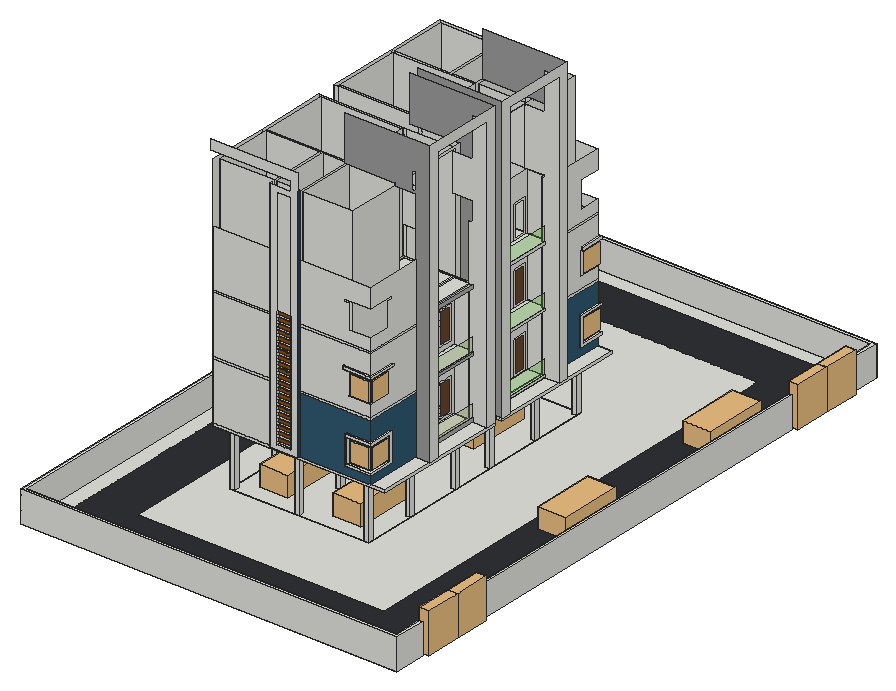
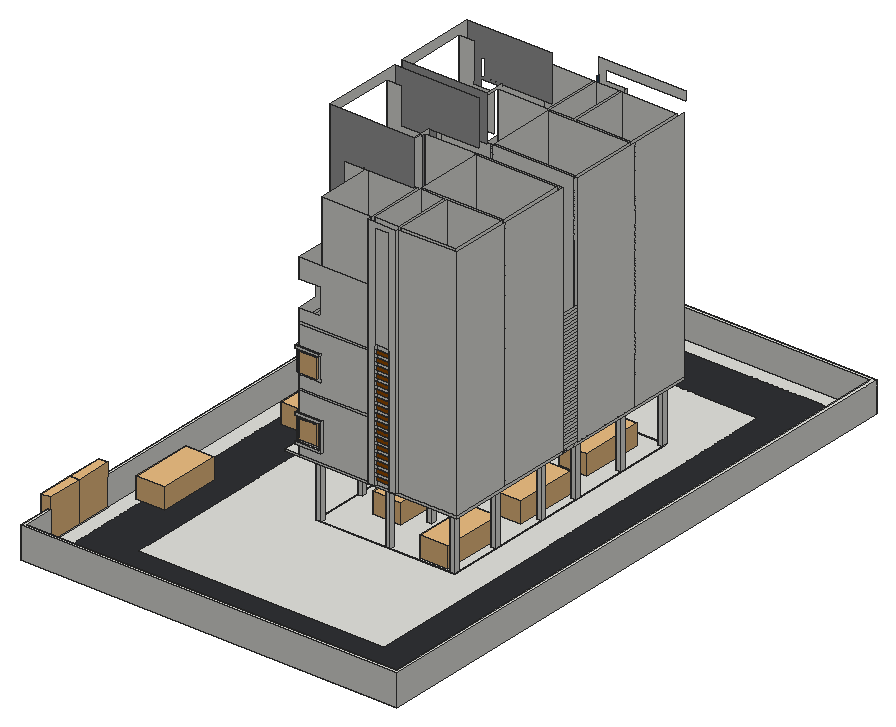
# SketchUp Ruby script. Lengths in inches.
U = 1.inch
M = Sketchup.active_model
def pt(a) = Geom::Point3d.new(a.map { |v| v * U })
def face(e, loops, mat)
  f = e.add_face(loops[0].map { |a| pt(a) })
  loops[1..].each { |l| e.add_face(l.map { |a| pt(a) }).erase! }
  f.material = f.back_material = mat if mat
  f
end
# faces: each face lists its corners as indices into pts; further lists are holes
def faces(e, pts, list, mat = nil) = list.each { |f| face(e, (f[0].is_a?(Array) ? f : [f]).map { |l| l.map { |i| pts[i] } }, mat) }
# xy, xz, yz: faces in a plane at the given z, y or x. An outline is a flat list of corners, or four numbers for a rectangle; further outlines are holes
def ring(l) = l.size == 4 ? [[l[0], l[1]], [l[2], l[1]], [l[2], l[3]], [l[0], l[3]]] : l.each_slice(2).to_a
def flat(e, list, mat, &to3) = list.each { |f| face(e, (f[0].is_a?(Array) ? f : [f]).map { |l| ring(l).map { |u, v| to3.(u, v) } }, mat) }
def xy(e, z, list, mat = nil) = flat(e, list, mat) { |x, y| [x, y, z] }
def xz(e, y, list, mat = nil) = flat(e, list, mat) { |x, z| [x, y, z] }
def yz(e, x, list, mat = nil) = flat(e, list, mat) { |y, z| [x, y, z] }
def lines(e, pts, list) = list.each { |a, b| e.add_line(pt(pts[a]), pt(pts[b])) }
# prism: a flat outline (further loops are holes) pulled along v
def prism(e, loops, v, mat = nil)
  f = face(e, loops, mat); d = Geom::Vector3d.new(v.map { |x| x * U })
  f.pushpull(f.normal.samedirection?(d) ? d.length : -d.length)
end
def box(e, o, s, mat = nil) = prism(e, [[o, [o[0] + s[0], o[1], o[2]], [o[0] + s[0], o[1] + s[1], o[2]], [o[0], o[1] + s[1], o[2]]]], [0, 0, s[2]], mat)
def at(x, y, z, deg = 0) = Geom::Transformation.translation(pt([x, y, z])) * Geom::Transformation.rotation(ORIGIN, Z_AXIS, deg.degrees)
def axes(o, x, y, z) = Geom::Transformation.new([*x, 0, *y, 0, *z, 0, *pt(o).to_a, 1])
def part(name) = M.definitions.add(name)
# library, detail: a bought-in or finely detailed component or shape, given as its bounding box
def library(name, o, s) = part(name).tap { |d| box(d.entities, o, s) }
def detail(e, o, s) = box(e.add_group.entities, o, s)
def put(e, d, t, mat = nil) = e.add_instance(d, t).tap { |i| i.material = mat if mat }
def group(e, t, mat = nil) = e.add_group.tap { |g| g.transformation = t; g.material = mat if mat }.entities
root = M.entities
M.materials.add("C07_Caramel_Shine").color = [153, 76, 0]
M.materials.add("Carpet_04_1K").color = [43, 65, 85]
M.materials.add("Glass_Basic_01").color = [173, 201, 98]
M.materials["Glass_Basic_01"].alpha = 0.25
M.materials.add("Glass_Basic_1").color = [130, 186, 66]
M.materials["Glass_Basic_1"].alpha = 0.25
M.materials.add("Glass_Basic_2").color = [93, 234, 42]
M.materials["Glass_Basic_2"].alpha = 0.25
M.materials.add("ThomThom - Buttons1").color = [48, 49, 53]
M.materials.add("ThomThom - Jumper1").color = [47, 89, 112]
M.materials.add("ThomThom - Waistcoat1").color = [155, 155, 155]
M.materials.add("ThomThom - Waistcoat2").color = [170, 170, 169]
M.materials.add("Wood_Veneer_15_1K").color = [103, 69, 45]
c1 = library("2016+Honda+Civic+LX+Sedan",[0.01,0.03,0.02],[16.17,34.46,10.62])
c2 = library("Ornamental gate leaf",[0,0,0],[161.42,42.43,280.3])
c3 = part("cong")
put(c3.entities,c2,axes([244.78,234.5625,0],[-1,0,0],[0,1,0],[0,0,1]))
put(c3.entities,c2,at(244.78,234.5625,0))
c4 = library("Group\#5",[0,0,0],[1.97,28.21,60])
xy(root,-12,[[[0,0,0,1506,948,1506,948,1421.02,939,1421.02,939,1241.02,948,1241.02,948,260.15,939,260.15,939,80.15,948,80.15,948,0],[240,360,588,1026]],[240,360,588,1026]])
xy(root,-6,[[[9,9,939,1497],[45,45,903,1461]],[[165,165,783,1341],[240,360,588,1026]],[240,360,588,1026]])
xy(root,-6,[[[45,45,903,1461],[165,165,783,1341]]],"ThomThom - Buttons1")
xy(root,66,[[0,0,948,0,948,80.15,939,80.15,939,9,9,9,9,1497,939,1497,939,1421.02,948,1421.02,948,1506,0,1506],[939,260.15,948,1241.02]])
xy(root,143.66,[[612,705,648,729],[612,885,648,909]])
xy(root,144,[[363,330,435,336],[[216,336,216,669,225,669,225,345,363,345,363,489,225,489,225,495,429,495,429,663,225,663,225,669,561,669,561,681,612,681,612,336],[435,495,555,663],[435,345,561,489],[369,345,429,489],[561,495,603,663]],[612,477,648,501],[612,657,648,681],[561,705,603,717],
  [555,723,561,891],[561,897,603,1041],[363,1050,381,1056],[417,1050,435,1056]])
xy(root,149.66,[[603,729,612,885]])
xy(root,155.71,[[381,1050,417,1053]])
xy(root,156,[[381,330,417,336]])
xy(root,163.125,[[381,333,417,336]])
xy(root,163.72,[[381,1050,417,1053]])
xy(root,168,[[552,330,558,336],[558,330,618,336],[612,336,618,337.15],[612,337.15,618,396],[612,990,618,1050],
  [551.39,1050,618,1056]])
xy(root,170.25,[[381,333,417,336]])
xy(root,172.65,[[381,1050,417,1053]])
xy(root,174,[[558,330,618,330,618,390,612,390,612,336,558,336],[612,996,612,1050,557.39,1050,557.39,1056,618,1056,618,996]])
xy(root,177.375,[[381,333,417,336]])
xy(root,181.57,[[381,1050,417,1053]])
xy(root,184.5,[[381,333,417,336]])
xy(root,190.5,[[381,1050,417,1053]])
xy(root,191.625,[[381,333,417,336]])
xy(root,198.75,[[381,333,417,336]])
xy(root,199.42,[[381,1050,417,1053]])
xy(root,205.875,[[381,333,417,336]])
xy(root,208.35,[[381,1050,417,1053]])
xy(root,213,[[381,333,417,336]])
xy(root,217.27,[[381,1050,417,1053]])
xy(root,220.125,[[381,333,417,336]])
xy(root,226.2,[[381,1050,417,1053]])
xy(root,227.25,[[381,333,417,336]])
xy(root,234,[[558,330,618,336],[612,336,618,390],[612,996,618,996,618,1056,557.39,1056,557.39,1050,612,1050]])
xy(root,234.375,[[381,333,417,336]])
xy(root,235.125,[[381,1050,417,1053]])
xy(root,240,[[552,330,618,330,618,396,612,396,612,336,552,336],[612,990,618,1050],[551.39,1050,618,1056]])
xy(root,241.5,[[381,333,417,336]])
xy(root,244.05,[[381,1050,417,1053]])
xy(root,248.625,[[381,333,417,336]])
xy(root,252.97,[[381,1050,417,1053]])
xy(root,255.75,[[381,333,417,336]])
xy(root,261.9,[[381,1050,417,1053]])
xy(root,262.875,[[381,333,417,336]])
xy(root,270,[[381,333,417,336]])
xy(root,270.82,[[381,1050,417,1053]])
xy(root,277.125,[[381,333,417,336]])
xy(root,279.75,[[381,1050,417,1053]])
xy(root,284.25,[[381,333,417,336]])
xy(root,288.67,[[381,1050,417,1053]])
xy(root,291.375,[[381,333,417,336]])
xy(root,293.66,[[435,723,555,891],[555,723,561,891],[561,723,603,723,603,729,612,729,612,885,603,885,603,891,561,891]])
xy(root,294,[[603,501,612,657]])
xy(root,297,[[435,495,555,501],[555,495,561,501],[561,495,603,501],[435,501,555,501.73],[555,501,561,501.73],
  [561,501,603,501.73],[435,501.73,555,657],[555,501.73,561,657],[561,501.73,603,657],[435,657,555,663],
  [555,657,561,663],[561,657,603,663]])
xy(root,297.6,[[381,1050,417,1053]])
xy(root,298.5,[[381,333,417,336]])
xy(root,299.66,[[435,723,555,891],[555,723,561,891],[561,723,561,891,603,891,603,885,612,885,612,729,603,729,603,723]])
xy(root,300,[[435,495,555,663],[555,495,561,663],[561,495,603,495,603,501,612,501,612,657,603,657,603,663,561,663],[603,495,612,501]])
xy(root,305.625,[[381,333,417,336]])
xy(root,306.52,[[381,1050,417,1053]])
xy(root,312.75,[[381,333,417,336]])
xy(root,315.45,[[381,1050,417,1053]])
xy(root,319.875,[[381,333,417,336]])
xy(root,324.375,[[381,1050,417,1053]])
xy(root,327,[[381,333,417,336]])
xy(root,333.3,[[381,1050,417,1053]])
xy(root,334.125,[[381,333,417,336]])
xy(root,341.25,[[381,333,417,336]])
xy(root,342.22,[[381,1050,417,1053]])
xy(root,348.375,[[381,333,417,336]])
xy(root,351.15,[[381,1050,417,1053]])
xy(root,355.5,[[381,333,417,336]])
xy(root,360.07,[[381,1050,417,1053]])
xy(root,362.625,[[381,333,417,336]])
xy(root,369,[[381,1050,417,1053]])
xy(root,369.75,[[381,333,417,336]])
xy(root,376.875,[[381,333,417,336]])
xy(root,377.92,[[381,1050,417,1053]])
xy(root,384,[[546,330,558,336],[558,330,612,336],[612,330,618,390],[381,333,417,336],[612,390,618,402],
  [612,996,618,1002],[612,1002,618,1056],[557.39,1050,564.01,1056],[564.01,1050,612,1056]])
xy(root,386.85,[[381,1050,417,1053]])
xy(root,390,[[546,330,618,330,618,402,612,402,612,336,546,336],[612,996,612,1050,557.39,1050,557.39,1056,618,1056,618,996]])
xy(root,391.125,[[381,333,417,336]])
xy(root,395.77,[[381,1050,417,1053]])
xy(root,398.25,[[381,333,417,336]])
xy(root,404.7,[[381,1050,417,1053]])
xy(root,405.375,[[381,333,417,336]])
xy(root,412.5,[[381,333,417,336]])
xy(root,413.625,[[381,1050,417,1053]])
xy(root,419.625,[[381,333,417,336]])
xy(root,422.55,[[381,1050,417,1053]])
xy(root,426.75,[[381,333,417,336]])
xy(root,431.47,[[381,1050,417,1053]])
xy(root,433.875,[[381,333,417,336]])
xy(root,440.4,[[381,1050,417,1053]])
xy(root,441,[[381,333,417,336]])
xy(root,443.66,[[435,723,555,891],[555,723,561,891],[561,723,603,723,603,729,612,729,612,885,603,885,603,891,561,891]])
xy(root,444,[[603,501,612,657]])
xy(root,448.125,[[381,333,417,336]])
xy(root,449.32,[[381,1050,417,1053]])
xy(root,449.66,[[435,723,555,891],[555,723,561,891],[561,723,561,891,603,891,603,885,612,885,612,729,603,729,603,723]])
xy(root,450,[[435,495,555,663],[555,495,561,663],[561,495,603,663]])
xz(root,0,[[0,-12,948,66]])
xz(root,9,[[9,-6,939,66]])
xz(root,80.15,[[939,-12,948,66]])
xz(root,260.15,[[939,-12,948,66]])
xz(root,330,[[[363,144,435,144,435,786,216,786,216,762,417,762,417,738,363,738],[381,156,417,726]],[552,168,618,168,618,174,558,174,558,234,618,234,618,240,552,240],[546,384,618,390]])
xz(root,333,[[381,163.125,417,170.25],[381,177.375,417,184.5],[381,191.625,417,198.75],[381,205.875,417,213],[381,220.125,417,227.25],
  [381,234.375,417,241.5],[381,248.625,417,255.75],[381,262.875,417,270],[381,277.125,417,284.25],[381,291.375,417,298.5],
  [381,305.625,417,312.75],[381,319.875,417,327],[381,334.125,417,341.25],[381,348.375,417,355.5],[381,362.625,417,369.75],
  [381,376.875,417,384],[381,391.125,417,398.25],[381,405.375,417,412.5],[381,419.625,417,426.75],[381,433.875,417,441],
  [381,448.125,417,455.25]],"C07_Caramel_Shine")
xz(root,336,[[216,144,363,288],[381,156,417,163.125],[381,170.25,417,177.375],[558,174,612,174,612,180,564,180,564,228,612,228,612,234,558,234],[564,180,612,228],
  [381,184.5,417,191.625],[381,198.75,417,205.875],[381,213,417,220.125],[381,227.25,417,234.375],[381,241.5,417,248.625],
  [381,255.75,417,262.875],[381,270,417,277.125],[381,284.25,417,291.375],[216,288,363,294],[435,288,612,294],
  [216,294,363,438],[435,294,612,294,612,324,558,324,558,384,546,384,546,390,612,390,612,438,435,438],[381,298.5,417,305.625],[381,312.75,417,319.875],[558,324,612,324,612,330,564,330,564,378,612,378,612,384,558,384],
  [381,327,417,334.125],[564,330,612,378],[381,341.25,417,348.375],[381,355.5,417,362.625],[381,369.75,417,376.875],
  [381,384,417,391.125],[381,398.25,417,405.375],[381,412.5,417,419.625],[381,426.75,417,433.875],[216,438,363,444],
  [435,438,612,444],[381,441,417,448.125],[216,444,363,588],[435,444,612,444,612,474,558,474,558,534,546,534,546,540,612,540,612,588,435,588]])
xz(root,336,[[435,144,612,144,612,168,552,168,552,240,612,240,612,288,435,288]],"ThomThom - Jumper1")
xz(root,345,[[225,144,363,738],[369,144,429,738],[435,144,561,738]])
xz(root,360,[[240,-12,588,-6]])
xz(root,390,[[612,174,618,234]])
xz(root,396,[[612,168,618,174],[612,174,618,234],[612,234,618,240]])
xz(root,402,[[612,384,618,390]])
xz(root,477,[[612,144,648,144,648,858,435,858,435,744,602.94,744,602.94,786,612,786,612,744,561,744,561,738,612,738]],"ThomThom - Waistcoat1")
xz(root,489,[[225,144,363,738],[369,144,429,738],[435,144,561,738]])
xz(root,495,[[225,144,429,738],[429,144,435,150],[435,144,555,297],[555,144,561,297],[561,144,603,297],
  [429,150,435,294],[429,294,435,300],[429,300,435,444],[435,300,555,450],[555,300,561,450],
  [561,300,603,450],[429,444,435,450],[429,450,435,594],[435,450,603,453]])
xz(root,501,[[612,144,612,150,603,150,603,294,612,294,612,300,603,300,603,444,612,444,612,453,603,453,603,594,612,594,612,642,561,642,561,738,613,738,613,744,612,744,612,834,648,834,648,144]])
xz(root,657,[[612,144,648,144,648,834,612,834,612,744,613,744,613,738,561,738,561,642,612,642,612,594,603,594,603,453,612,453,612,444,603,444,603,300,612,300,612,294,603,294,603,150,612,150]])
xz(root,663,[[225,144,429,738],[435,144,555,297],[561,144,603,297],[435,297,555,300],[555,297,561,300],
  [435,300,555,450],[561,300,603,450],[435,450,555,453],[555,450,561,453],[561,450,603,453]])
xz(root,669,[[216,144,225,738],[225,144,429,738],[429,144,435,738],[435,144,561,738]])
xz(root,681,[[561,144,561,744,435,744,435,858,648,858,648,144]],"ThomThom - Waistcoat1")
xz(root,705,[[612,143.66,612,144,561,144,561,744,435,744,435,858,648,858,648,143.66]],"ThomThom - Waistcoat1")
xz(root,717,[[216,144,225,738],[225,144,429,738],[429,144,435,738],[435,144,561,738]])
xz(root,723,[[225,144,429,738],[435,144,555,293.66],[555,144,561,293.66],[561,144,603,293.66],[435,293.66,603,299.66],
  [435,299.66,555,443.66],[555,299.66,561,443.66],[561,299.66,603,443.66],[435,443.66,603,449.66],[435,449.66,555,593.66],
  [555,449.66,561,593.66],[561,449.66,603,593.66]])
xz(root,729,[[612,143.66,648,143.66,648,834,612,834,612,743.66,561,743.66,561,599.66,612,599.66,612,593.66,603,593.66,603,449.66,612,449.66,612,443.66,603,443.66,603,299.66,612,299.66,612,293.66,603,293.66,603,149.66,612,149.66],[603,293.66,612,299.66],[603,443.66,612,449.66]])
xz(root,885,[[612,143.66,612,149.66,603,149.66,603,293.66,612,293.66,612,299.66,603,299.66,603,443.66,612,443.66,612,449.66,603,449.66,603,593.66,612,593.66,612,599.66,561,599.66,561,743.66,612,743.66,612,834,648,834,648,143.66],[603,293.66,612,299.66],[603,443.66,612,449.66]])
xz(root,891,[[225,144,429,738],[429,144,435,150],[435,144,555,293.66],[561,144,603,293.66],[429,150,435,294],
  [435,293.66,555,299.43],[555,293.66,561,299.43],[561,293.66,603,299.43],[429,294,435,300],[435,299.43,555,299.66],
  [555,299.43,561,299.66],[561,299.43,603,299.66],[435,299.66,555,443.66],[561,299.66,603,443.66],[429,300,435,444],
  [435,443.66,555,449.66],[555,443.66,561,449.66],[561,443.66,603,449.66],[429,444,435,450],[435,449.66,555,593.66],
  [561,449.66,603,593.66],[429,450,435,594]])
xz(root,897,[[225,144,363,738],[369,144,429,738],[435,144,561,738]])
xz(root,909,[[612,143.66,648,143.66,648,858,435,858,435,744,612,744]],"ThomThom - Waistcoat1")
xz(root,990,[[612,168,618,240]])
xz(root,996,[[612,174,618,234],[612,384,618,390]])
xz(root,1026,[[240,-12,588,-6]])
xz(root,1041,[[225,144,363,738],[369,144,429,738],[435,144,561,738]])
xz(root,1050,[[216,144,363,738],[381,144,417,155.71],[435,144,612,144,612,168,551.39,168,551.39,240,612,240,612,288,435,288],[381,163.72,417,172.65],[557.39,174,612,174,612,180,564.01,180,564.01,228,612,228,612,234,557.39,234],
  [564.01,180,612,228],[381,181.57,417,190.5],[381,199.42,417,208.35],[381,217.27,417,226.2],[381,235.125,417,244.05],
  [381,252.97,417,261.9],[381,270.82,417,279.75],[435,288,612,294],[381,288.67,417,297.6],[435,294,612,294,612,324,557.39,324,557.39,390,612,390,612,438,435,438],
  [381,306.52,417,315.45],[557.39,324,612,324,612,330,564.01,330,564.01,378,612,378,612,384,557.39,384],[381,324.375,417,333.3],[564.01,330,612,378],[381,342.22,417,351.15],
  [381,360.07,417,369],[381,377.92,417,386.85],[381,395.77,417,404.7],[381,413.625,417,422.55],[381,431.47,417,440.4],
  [435,438,612,444],[435,444,612,444,612,474,557.39,474,557.39,540,612,540,612,588,435,588],[381,449.32,417,458.25]])
xz(root,1053,[[381,155.71,417,163.72],[381,172.65,417,181.57],[381,190.5,417,199.42],[381,208.35,417,217.27],[381,226.2,417,235.125],
  [381,244.05,417,252.97],[381,261.9,417,270.82],[381,279.75,417,288.67],[381,297.6,417,306.52],[381,315.45,417,324.375],
  [381,333.3,417,342.22],[381,351.15,417,360.07],[381,369,417,377.92],[381,386.85,417,395.77],[381,404.7,417,413.625],
  [381,422.55,417,431.47],[381,440.4,417,449.32]],"C07_Caramel_Shine")
xz(root,1056,[[363,144,381,144,381,726,417,726,417,144,435,144,435,738,363,738],[551.39,168,618,168,618,174,557.39,174,557.39,234,618,234,618,240,551.39,240],[557.39,384,618,390]])
xz(root,1241.02,[[939,-12,948,66]])
xz(root,1421.02,[[939,-12,948,66]])
xz(root,1497,[[9,-6,939,66]])
xz(root,1506,[[0,-12,948,66]])
yz(root,0,[[0,-12,1506,66]])
yz(root,9,[[9,-6,1497,66]])
yz(root,216,[[669,138,717,145.5],[336,144,489,738],[489,144,669,738],[717,144,897,738],[897,144,1050,738],
  [669,145.5,717,153],[669,153,717,160.5],[669,160.5,717,168],[669,168,717,175.5],[669,175.5,717,183],
  [669,183,717,190.5],[669,190.5,717,198],[669,198,717,205.5],[669,205.5,717,213],[669,213,717,220.5],
  [669,220.5,717,228],[669,228,717,235.5],[669,235.5,717,243],[669,243,717,250.5],[669,250.5,717,258],
  [669,258,717,265.5],[669,265.5,717,273],[669,273,717,280.5],[669,280.5,717,288],[669,288,717,295.5],
  [669,295.5,717,303],[669,303,717,310.5],[669,310.5,717,318],[669,318,717,325.5],[669,325.5,717,333],
  [669,333,717,340.5],[669,340.5,717,348],[669,348,717,355.5],[669,355.5,717,363],[669,363,717,370.5],
  [669,370.5,717,378],[669,378,717,385.5],[669,385.5,717,393],[669,393,717,400.5],[669,400.5,717,408],
  [669,408,717,415.5],[669,415.5,717,423],[669,423,717,430.5],[669,430.5,717,438],[669,438,717,445.5],
  [669,445.5,717,453]])
yz(root,225,[[345,144,489,738],[489,144,495,150],[495,144,663,738],[663,144,669,150],[717,144,723,150],
  [723,144,891,738],[891,144,897,150],[897,144,1041,738],[489,150,495,294],[663,150,669,294],
  [717,150,723,294],[891,150,897,294],[489,294,495,300],[663,294,669,300],[717,294,723,300],
  [891,294,897,300],[489,300,495,444],[663,300,669,444],[717,300,723,444],[891,300,897,444],
  [489,444,495,450],[663,444,669,450],[717,444,723,450],[891,444,897,450],[489,450,495,594],
  [663,450,669,594],[717,450,723,594],[891,450,897,594]])
yz(root,240,[[360,-12,720,-6],[720,-12,1026,-6]])
yz(root,363,[[330,144,336,738],[345,144,489,738],[897,144,1041,738],[1050,144,1056,738]])
yz(root,369,[[345,144,489,738],[897,144,1041,738]])
yz(root,381,[[1050,144,1050,155.71,1053,155.71,1053,163.72,1056,163.72,1056,144],[330,156,336,163.125],[330,163.125,333,170.25],[1050,163.72,1056,172.65],[330,170.25,336,177.375],
  [1053,172.65,1056,181.57],[330,177.375,333,184.5],[1050,181.57,1056,190.5],[330,184.5,336,191.625],[1053,190.5,1056,199.42],
  [330,191.625,333,198.75],[330,198.75,336,205.875],[1050,199.42,1056,208.35],[330,205.875,333,213],[1053,208.35,1056,217.27],
  [330,213,336,220.125],[1050,217.27,1056,226.2],[330,220.125,333,227.25],[1053,226.2,1056,235.125],[330,227.25,336,234.375],
  [330,234.375,333,241.5],[1050,235.125,1056,244.05],[330,241.5,336,248.625],[1053,244.05,1056,252.97],[330,248.625,333,255.75],
  [1050,252.97,1056,261.9],[330,255.75,336,262.875],[1053,261.9,1056,270.82],[330,262.875,333,270],[330,270,336,277.125],
  [1050,270.82,1056,279.75],[330,277.125,333,284.25],[1053,279.75,1056,288.67],[330,284.25,336,291.375],[1050,288.67,1056,297.6],
  [330,291.375,333,298.5],[1053,297.6,1056,306.52],[330,298.5,336,305.625],[330,305.625,333,312.75],[1050,306.52,1056,315.45],
  [330,312.75,336,319.875],[1053,315.45,1056,324.375],[330,319.875,333,327],[1050,324.375,1056,333.3],[330,327,336,334.125],
  [1053,333.3,1056,342.22],[330,334.125,333,341.25],[330,341.25,336,348.375],[1050,342.22,1056,351.15],[330,348.375,333,355.5],
  [1053,351.15,1056,360.07],[330,355.5,336,362.625],[1050,360.07,1056,369],[330,362.625,333,369.75],[1053,369,1056,377.92],
  [330,369.75,336,376.875],[330,376.875,333,384],[1050,377.92,1056,386.85],[330,384,336,391.125],[1053,386.85,1056,395.77],
  [330,391.125,333,398.25],[1050,395.77,1056,404.7],[330,398.25,336,405.375],[1053,404.7,1056,413.625],[330,405.375,333,412.5],
  [330,412.5,336,419.625],[1050,413.625,1056,422.55],[330,419.625,333,426.75],[1053,422.55,1056,431.47],[330,426.75,336,433.875],
  [1050,431.47,1056,440.4],[330,433.875,333,441],[1053,440.4,1056,449.32],[330,441,336,448.125],[330,448.125,333,455.25],
  [1050,449.32,1056,458.25]])
yz(root,417,[[1050,144,1056,144,1056,163.72,1053,163.72,1053,155.71,1050,155.71],[330,156,336,163.125],[330,163.125,333,170.25],[1050,163.72,1056,172.65],[330,170.25,336,177.375],
  [1053,172.65,1056,181.57],[330,177.375,333,184.5],[1050,181.57,1056,190.5],[330,184.5,336,191.625],[1053,190.5,1056,199.42],
  [330,191.625,333,198.75],[330,198.75,336,205.875],[1050,199.42,1056,208.35],[330,205.875,333,213],[1053,208.35,1056,217.27],
  [330,213,336,220.125],[1050,217.27,1056,226.2],[330,220.125,333,227.25],[1053,226.2,1056,235.125],[330,227.25,336,234.375],
  [330,234.375,333,241.5],[1050,235.125,1056,244.05],[330,241.5,336,248.625],[1053,244.05,1056,252.97],[330,248.625,333,255.75],
  [1050,252.97,1056,261.9],[330,255.75,336,262.875],[1053,261.9,1056,270.82],[330,262.875,333,270],[330,270,336,277.125],
  [1050,270.82,1056,279.75],[330,277.125,333,284.25],[1053,279.75,1056,288.67],[330,284.25,336,291.375],[1050,288.67,1056,297.6],
  [330,291.375,333,298.5],[1053,297.6,1056,306.52],[330,298.5,336,305.625],[330,305.625,333,312.75],[1050,306.52,1056,315.45],
  [330,312.75,336,319.875],[1053,315.45,1056,324.375],[330,319.875,333,327],[1050,324.375,1056,333.3],[330,327,336,334.125],
  [1053,333.3,1056,342.22],[330,334.125,333,341.25],[330,341.25,336,348.375],[1050,342.22,1056,351.15],[330,348.375,333,355.5],
  [1053,351.15,1056,360.07],[330,355.5,336,362.625],[1050,360.07,1056,369],[330,362.625,333,369.75],[1053,369,1056,377.92],
  [330,369.75,336,376.875],[330,376.875,333,384],[1050,377.92,1056,386.85],[330,384,336,391.125],[1053,386.85,1056,395.77],
  [330,391.125,333,398.25],[1050,395.77,1056,404.7],[330,398.25,336,405.375],[1053,404.7,1056,413.625],[330,405.375,333,412.5],
  [330,412.5,336,419.625],[1050,413.625,1056,422.55],[330,419.625,333,426.75],[1053,422.55,1056,431.47],[330,426.75,336,433.875],
  [1050,431.47,1056,440.4],[330,433.875,333,441],[1053,440.4,1056,449.32],[330,441,336,448.125],[330,448.125,333,455.25],
  [1050,449.32,1056,458.25]])
yz(root,429,[[345,144,489,738],[495,144,663,738],[723,144,891,738],[897,144,1041,738]])
yz(root,435,[[345,144,489,738],[495,144,663,297],[723,144,891,293.66],[897,144,1041,738],[1050,144,1056,738],
  [495,297,663,300],[723,299.66,891,443.66],[495,300,663,450],[723,449.66,891,593.66],[495,450,663,453]])
yz(root,435,[[330,144,336,744]],"Carpet_04_1K")
yz(root,546,[[330,384,336,390]])
yz(root,551.39,[[1050,168,1056,240]])
yz(root,552,[[330,168,336,174],[330,174,336,234],[330,234,336,240]])
yz(root,557.39,[[1050,174,1056,234],[1050,384,1056,390]])
yz(root,558,[[330,174,336,234]])
yz(root,561,[[345,144,345,738,477,738,477,744,681,744,681,144,669,144,669,738,489,738,489,144],[[495,144,663,297],[615,148.61,651,232.61],[543,181.61,591,229.61]],[705,144,717,144,717,738,729,738,729,743.66,885,743.66,885,738,897,738,897,144,1041,144,1041,738,909,738,909,744,705,744],[[723,144,723,293.66,891,293.66,891,144,885,144,885,228,849,228,849,144],[777,180,825,228]],[[849,144,885,228],[852,147,882,225]],
  [[615,148.61,651,232.61],[618,151.61,648,229.61]],[[777,180,825,228],[780,183,822,225]],[[543,181.61,591,229.61],[546,184.61,588,226.61]],[[723,299.66,723,443.66,891,443.66,891,299.66,885,299.66,885,383.66,849,383.66,849,299.66],[777,335.66,825,383.66]],[[849,299.66,885,383.66],[852,302.66,882,380.66]],
  [[495,300,663,450],[615,311.08,651,395.08],[543,347.08,591,395.08]],[[615,311.08,651,395.08],[618,314.08,648,392.08]],[[777,335.66,825,383.66],[780,338.66,822,380.66]],[[543,347.08,591,395.08],[546,350.08,588,392.08]],[[723,449.66,723,593.66,891,593.66,891,449.66,885,449.66,885,533.66,849,533.66,849,449.66],[777,485.66,825,533.66]],
  [[849,449.66,885,533.66],[852,452.66,882,530.66]]])
yz(root,561,[[852,147,882,225],[618,151.61,648,229.61],[852,302.66,882,380.66],[618,314.08,648,392.08]],"Wood_Veneer_15_1K")
yz(root,588,[[360,-12,1026,-6]])
yz(root,603,[[[495,144,663,297],[501,150,657,294]],[723,144,891,144,891,293.66,885,293.66,885,149.66,729,149.66,729,293.66,723,293.66],[723,293.66,729,299.66],[885,293.66,891,299.43],[885,299.43,891,299.66],
  [723,299.66,729,443.66],[885,299.66,891,443.66],[495,300,495,450,663,450,663,300,657,300,657,444,501,444,501,300],[723,443.66,729,449.66],[885,443.66,891,449.66],
  [723,449.66,729,593.66],[885,449.66,891,593.66],[495,450,657,453],[657,450,663,453]])
yz(root,612,[[705,143.66,729,144],[729,143.66,885,144],[885,143.66,909,144],[729,144,885,149.66],[336,174,390,174,390,234,336,234,336,228,384,228,384,180,336,180],
  [996,174,996,234,1050,234,1050,228,1002,228,1002,180,1050,180,1050,174],[336,180,384,228],[1002,180,1050,228],[336,288,477,294],[909,288,1050,294],
  [729,293.66,885,299.66],[336,294,477,294,477,438,336,438,336,390,402,390,402,384,390,384,390,324,336,324],[909,294,909,438,1050,438,1050,390,996,390,996,324,1050,324,1050,294],[336,324,390,324,390,384,336,384,336,378,384,378,384,330,336,330],[996,324,996,384,1050,384,1050,378,1002,378,1002,330,1050,330,1050,324],
  [336,330,384,378],[1002,330,1050,378],[336,438,477,444],[909,438,1050,444],[729,443.66,885,449.66],
  [336,444,477,444,477,588,336,588,336,540,402,540,402,534,390,534,390,474,336,474],[909,444,909,588,1050,588,1050,540,996,540,996,474,1050,474,1050,444]])
yz(root,612,[[501,153,657,186]],"Glass_Basic_01")
yz(root,612,[[501,303,657,336]],"Glass_Basic_1")
yz(root,612,[[729,149.66,885,185.66],[729,299.66,885,335.66],[729,449.66,885,485.66]],"Glass_Basic_2")
yz(root,612,[[336,144,477,144,477,288,336,288,336,240,396,240,396,168,336,168],[909,144,909,288,1050,288,1050,240,990,240,990,168,1050,168,1050,144]],"ThomThom - Jumper1")
yz(root,612,[[501,144,657,153],[501,294,657,300],[501,300,657,303],[501,444,657,453]],"ThomThom - Waistcoat2")
yz(root,618,[[330,168,396,168,396,240,330,240,330,234,390,234,390,174,330,174],[990,168,990,240,1056,240,1056,234,996,234,996,174,1056,174,1056,168],[330,384,402,390],[996,384,1056,390]])
yz(root,648,[[705,143.66,705,858,909,858,909,143.66,885,143.66,885,834,729,834,729,143.66],[477,144,501,144,501,834,657,834,657,144,681,144,681,858,477,858]])
yz(root,939,[[80.15,-12,260.15,-6],[1241.02,-12,1421.02,-6],[9,-6,80.15,66],[260.15,-6,1241.02,66],[1421.02,-6,1497,66]])
yz(root,948,[[0,-12,80.15,66],[260.15,-12,1241.02,66],[1421.02,-12,1506,66]])
p = [[561,489,144],[612,489,144],[603,489,150],[612,489,150],[603,489,294],[612,489,294],
  [603,489,300],[612,489,300],[603,663,444],[612,663,444],[612,409.46,240],[558,336,240],
  [603,897,144],[612,897,144],[603,897,150],[612,897,150],[603,897,294],[612,897,294],
  [603,897,300],[612,897,300],[603,723,444],[612,723,444]]
lines(root,p,[[0,1],[2,3],[4,5],[6,7],[8,9],[10,11],[12,13],[14,15],[16,17],[18,19],[20,21]])
put(root,c1,axes([811.18,612.07,-8.65],[4.4275,0,0],[0,4.5484,0],[0,0,4.833]))
g1 = group(root,at(216,717,138))
xy(g1,-144,[[24,24,36,36],[186,24,198,36],[360,24,372,36],[24,166.5,36,178.5],[186,166.5,198,178.5],
  [360,166.5,372,178.5],[24,297,36,309],[186,297,198,309],[360,297,372,309]])
xy(g1,0,[[[0,-12,432,333],[24,24,372,309]],[36,24,186,36],[198,24,360,36],[24,36,36,166.5],[36,36,186,166.5],
  [186,36,198,166.5],[198,36,360,166.5],[360,36,372,166.5],[36,166.5,186,178.5],[198,166.5,360,178.5],
  [24,178.5,36,297],[36,178.5,186,297],[186,178.5,198,297],[198,178.5,360,297],[360,178.5,372,297],
  [36,297,186,309],[198,297,360,309]])
xy(g1,6,[[0,-12,432,333]])
xz(g1,-12,[[0,0,432,6]])
xz(g1,24,[[24,-144,36,0],[186,-144,198,0],[360,-144,372,0]])
xz(g1,36,[[24,-144,36,0],[186,-144,198,0],[360,-144,372,0]])
xz(g1,166.5,[[24,-144,36,0],[186,-144,198,0],[360,-144,372,0]])
xz(g1,178.5,[[24,-144,36,0],[186,-144,198,0],[360,-144,372,0]])
xz(g1,297,[[24,-144,36,0],[186,-144,198,0],[360,-144,372,0]])
xz(g1,309,[[24,-144,36,0],[186,-144,198,0],[360,-144,372,0]])
xz(g1,333,[[0,0,432,6]])
yz(g1,0,[[-12,0,333,6]])
yz(g1,24,[[24,-144,36,0],[166.5,-144,178.5,0],[297,-144,309,0]])
yz(g1,36,[[24,-144,36,0],[166.5,-144,178.5,0],[297,-144,309,0]])
yz(g1,186,[[24,-144,36,0],[166.5,-144,178.5,0],[297,-144,309,0]])
yz(g1,198,[[24,-144,36,0],[166.5,-144,178.5,0],[297,-144,309,0]])
yz(g1,360,[[24,-144,36,0],[166.5,-144,178.5,0],[297,-144,309,0]])
yz(g1,372,[[24,-144,36,0],[166.5,-144,178.5,0],[297,-144,309,0]])
yz(g1,432,[[-12,0,333,6]])
put(root,c1,axes([281.68,400.375,-6.11],[4.4275,0,0],[0,4.5484,0],[0,0,4.833]))
g2 = group(root,at(216,336,-6))
xy(g2,0,[[24,24,36,36],[186,24,198,36],[360,24,372,36],[24,154.5,36,166.5],[186,154.5,198,166.5],
  [360,154.5,372,166.5],[24,297,36,309],[186,297,198,309],[360,297,372,309]])
xy(g2,144,[[[0,0,432,345],[24,24,372,309]],[36,24,186,36],[198,24,360,36],[24,36,36,154.5],[36,36,186,154.5],
  [186,36,198,154.5],[198,36,360,154.5],[360,36,372,154.5],[36,154.5,186,166.5],[198,154.5,360,166.5],
  [24,166.5,36,297],[36,166.5,186,297],[186,166.5,186,297,198,297,198,309,360,309,360,297,372,297,372,166.5,360,166.5,360,296.55,198,296.55,198,166.5],[198,166.5,360,296.55],[36,297,186,309]])
xy(g2,150,[[0,0,432,345]])
xz(g2,0,[[0,144,432,150]])
xz(g2,24,[[24,0,36,144],[186,0,198,144],[360,0,372,144]])
xz(g2,36,[[24,0,36,144],[186,0,198,144],[360,0,372,144]])
xz(g2,154.5,[[24,0,36,144],[186,0,198,144],[360,0,372,144]])
xz(g2,166.5,[[24,0,36,144],[186,0,198,144],[360,0,372,144]])
xz(g2,297,[[24,0,36,144],[186,0,198,144],[360,0,372,144]])
xz(g2,309,[[24,0,36,144],[186,0,198,144],[360,0,372,144]])
xz(g2,345,[[0,144,432,150]])
yz(g2,0,[[0,144,345,150]])
yz(g2,24,[[24,0,36,144],[154.5,0,166.5,144],[297,0,309,144]])
yz(g2,36,[[24,0,36,144],[154.5,0,166.5,144],[297,0,309,144]])
yz(g2,186,[[24,0,36,144],[154.5,0,166.5,144],[297,0,309,144]])
yz(g2,198,[[24,0,36,144],[154.5,0,166.5,144],[297,0,309,144]])
yz(g2,360,[[24,0,36,144],[154.5,0,166.5,144],[297,0,309,144]])
yz(g2,372,[[24,0,36,144],[154.5,0,166.5,144],[297,0,309,144]])
yz(g2,432,[[0,144,345,150]])
p = [[24,154.5,0],[24,36,0],[24,297,0],[24,166.5,0],[372,690,0],[24,690,0],
  [24,309,0],[198,24,0],[360,24,0],[372,36,0],[372,154.5,0],[36,24,0],
  [186,24,0],[372,166.5,0],[372,297,0],[372,309,0]]
lines(g2,p,[[0,1],[2,3],[4,5],[5,6],[7,8],[9,10],[11,12],[13,14],[15,4]])
put(root,c1,axes([263.92,631.16,-6.11],[4.4275,0,0],[0,4.5484,0],[0,0,4.833]))
put(root,c1,axes([464.82,401.21,-6.11],[4.4275,0,0],[0,4.5484,0],[0,0,4.833]))
put(root,c1,axes([262.4,861.23,-6.11],[4.4275,0,0],[0,4.5484,0],[0,0,4.833]))
put(root,c3,axes([1096.89,33.65,-6],[0,0.5578,0],[-0.57,0,0],[0,0,0.36049]))
put(root,c1,axes([443.87,781.51,-6.11],[4.4275,0,0],[0,4.5484,0],[0,0,4.833]))
put(root,c3,axes([1096.89,1194.53,-6],[0,0.5578,0],[-0.57,0,0],[0,0,0.36049]))
put(root,c1,axes([832.59,1040.56,5.23],[4.4275,0,0],[0,4.5484,0],[0,0,4.833]))
put(root,c4,axes([616.44,1050,179.94],[-2.50681,0,0],[0,-1.70151,0],[0,0,0.801]))
put(root,c4,axes([564,331.56,179.94],[0,2.50681,0],[1.70151,0,0],[0,0,0.801]))
put(root,c4,axes([616.93,336,180],[-2.50681,0,0],[0,1.70151,0],[0,0,0.801]))
put(root,c4,axes([564.04,1052.45,180.01],[0,-1.3838,0],[1.7,0,0],[0,0,0.7998]))
put(root,c4,axes([565.44,822,183],[-2.50681,0,0],[0,-1.48882,0],[0,0,0.70007]))
put(root,c4,axes([565.93,546,184.61],[-2.50681,0,0],[0,1.48882,0],[0,0,0.70007]))
put(root,c4,axes([616.44,1050,329.94],[-2.50681,0,0],[0,-1.70151,0],[0,0,0.801]))
put(root,c4,axes([564,331.56,329.94],[0,2.50681,0],[1.70151,0,0],[0,0,0.801]))
put(root,c4,axes([616.93,336,330],[-2.50681,0,0],[0,1.70151,0],[0,0,0.801]))
put(root,c4,axes([564.04,1052.45,330.01],[0,-1.3838,0],[1.7,0,0],[0,0,0.7998]))
put(root,c4,axes([565.44,822,338.66],[-2.50681,0,0],[0,-1.48882,0],[0,0,0.70007]))
put(root,c4,axes([565.93,546,350.08],[-2.50681,0,0],[0,1.48882,0],[0,0,0.70007]))
